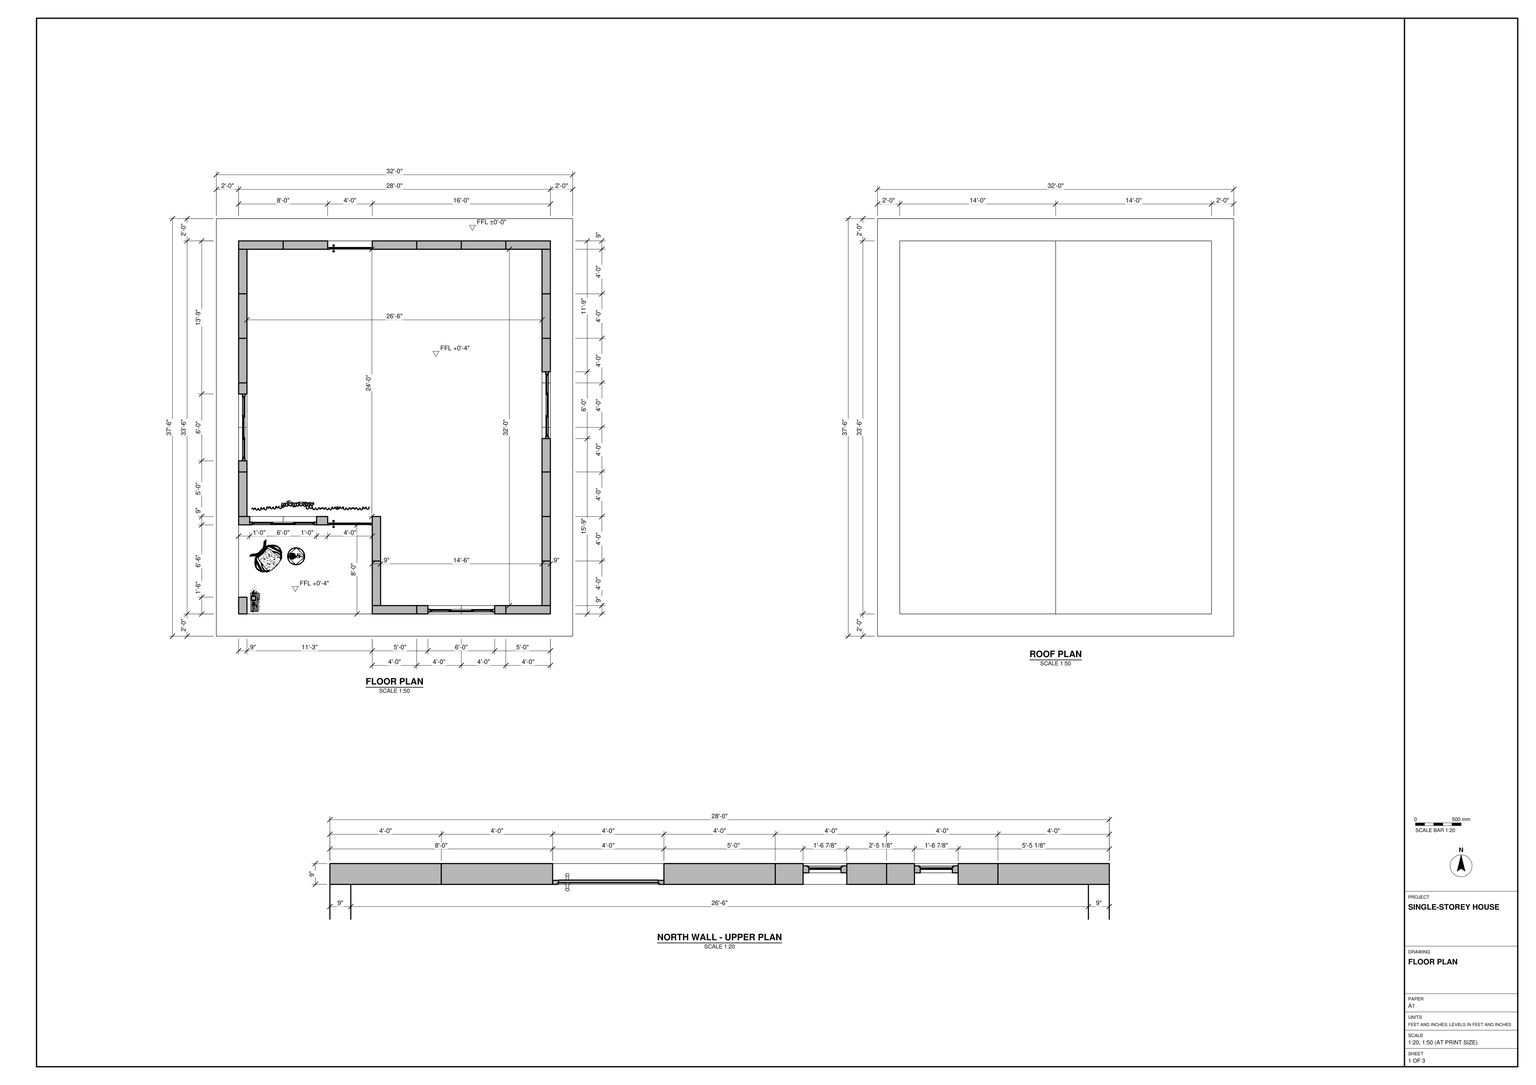
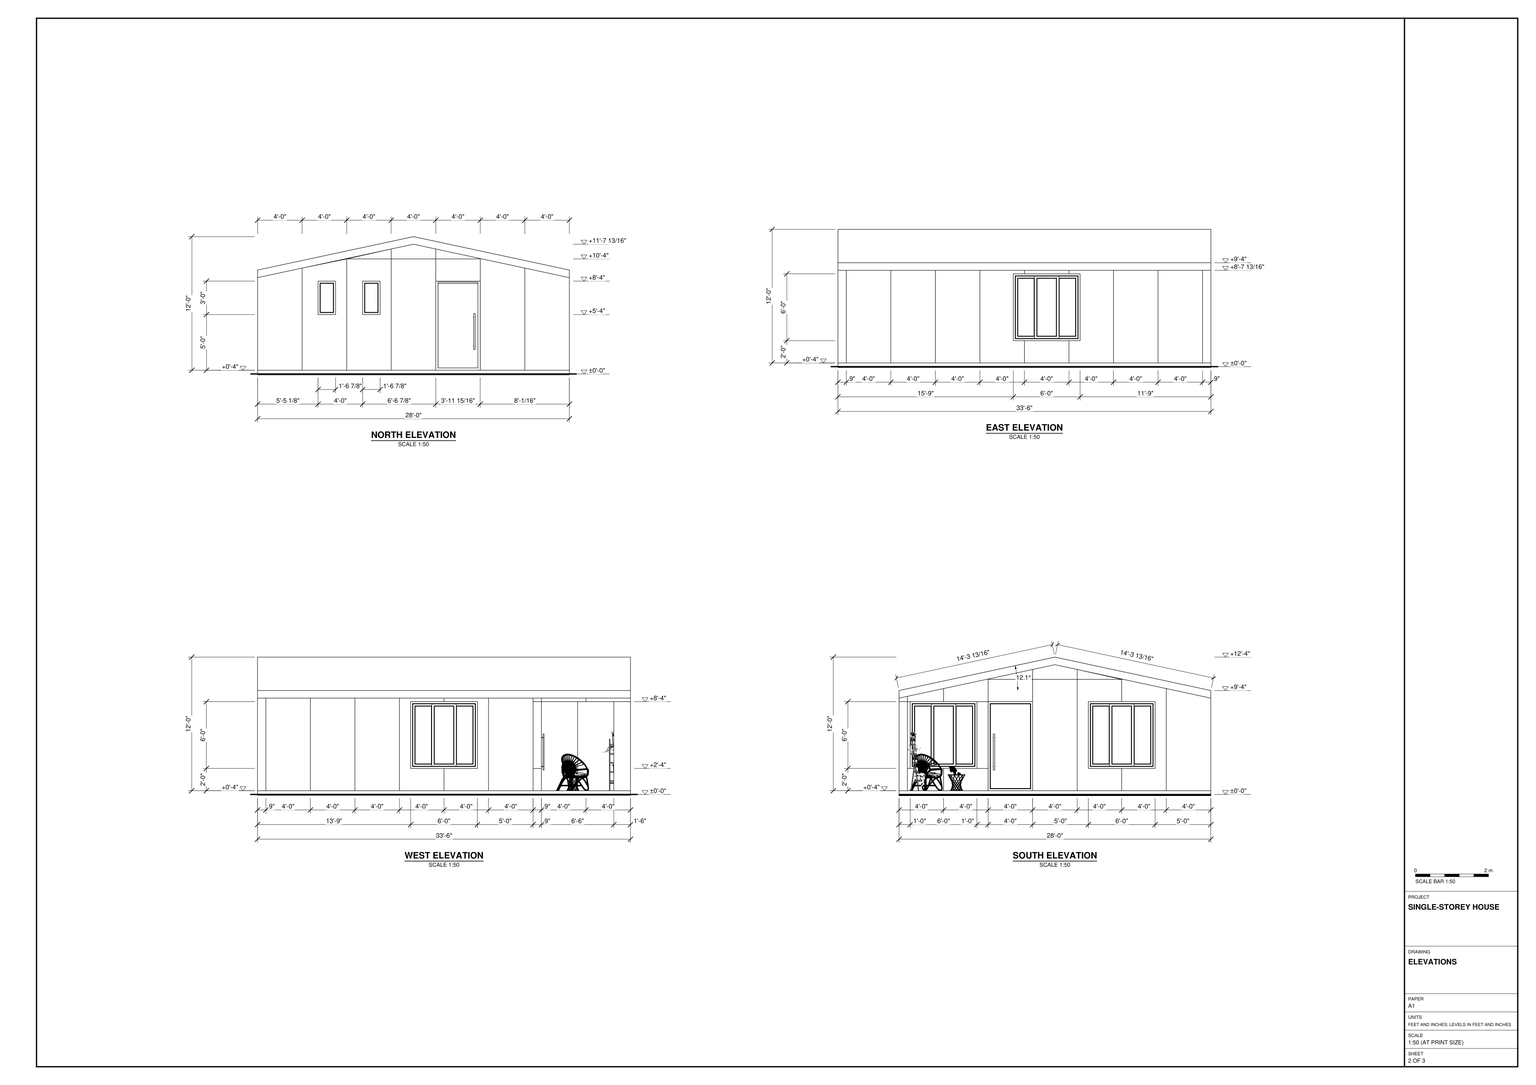
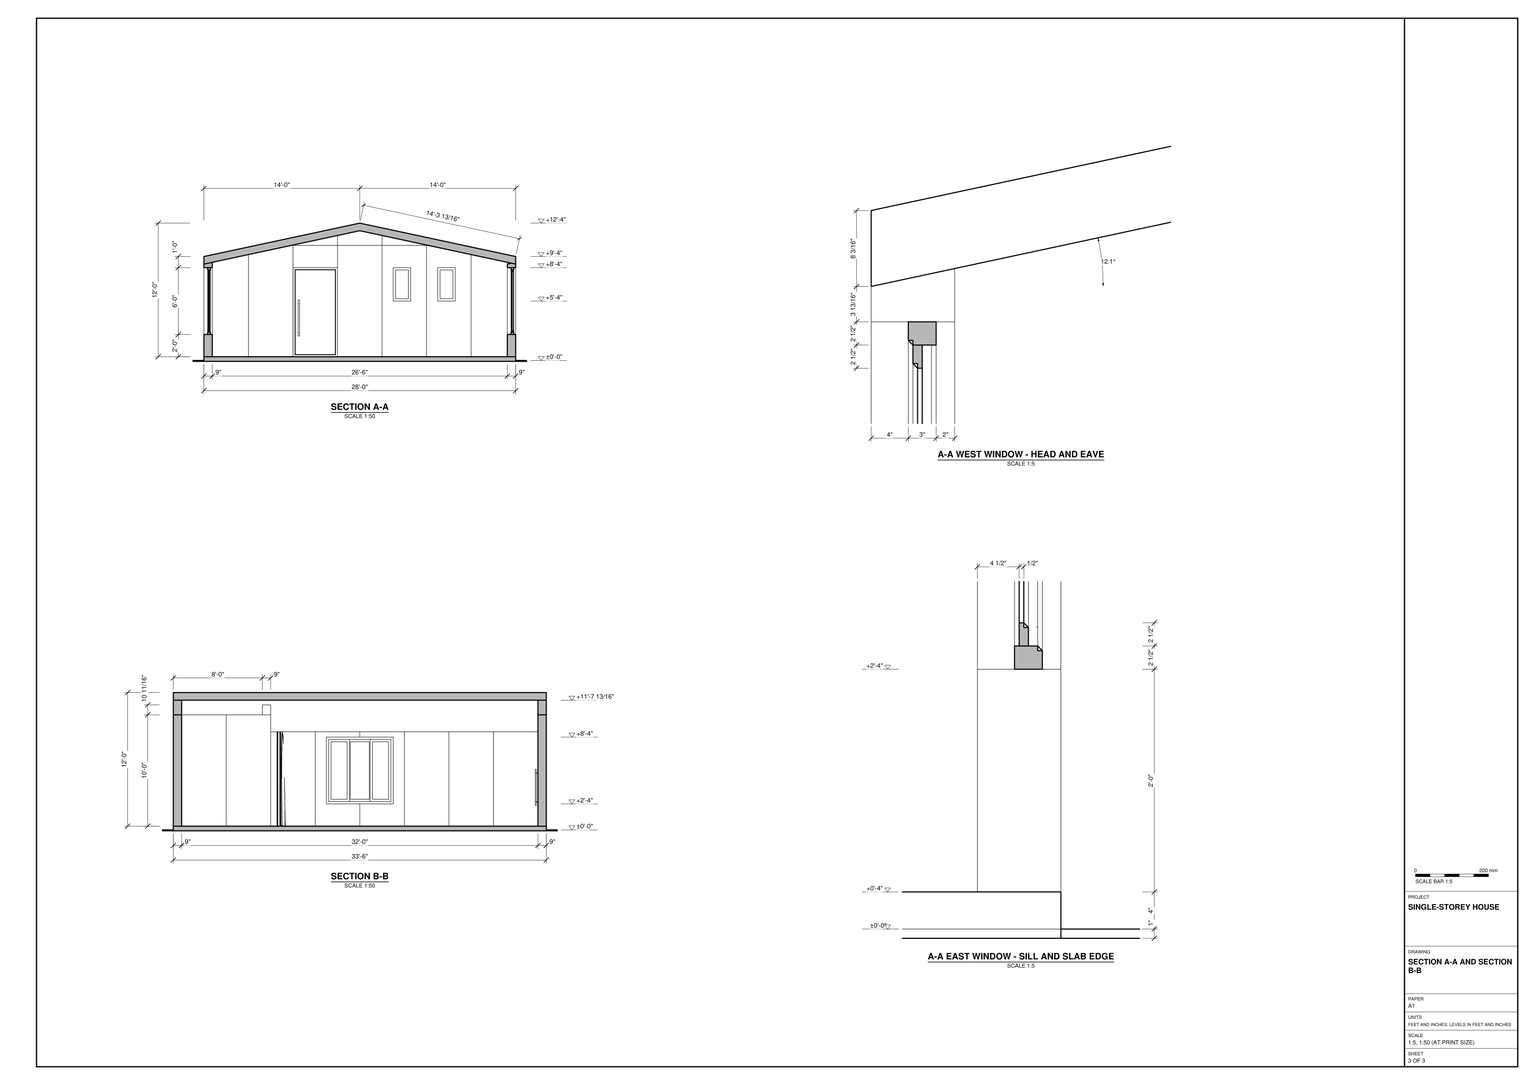
Build the house in SketchUp from task_files/diagram_01.pdf. Work in feet and inches. The complete model, including the surrounding ground, measures 128'-0" along X, 133'-6" along Y and 12'-5" along Z. Use ±0'-0" as the ground datum for the single storey. Set the finished floor and porch surface at +0'-4".

Set out the house within a 28'-0" by 33'-6" footprint. Follow the floor plan for the 9" walls, the open interior and the porch recessed into the southwest corner. Include the porch corner post and the seating and small table shown there. Model the slab edge and the vertical wall panel joints shown in the sections and elevations. Fit the north door beside the two narrow windows. On the south side, distinguish the door and window in the recessed wall from the window in the projecting wall. Use the sections to set the window frames, heads and sills into the side walls.

Carry the gable roof across the porch, with equal slopes meeting at a north–south ridge. Keep walls, slab, roof and each furniture or joinery piece in separate groups or components, and use components for repeated parts. Decor and loose items may be any suitable library components, for example from 3D Warehouse. Save one SketchUp model as output_files/single_storey_gabled_house_with_a_recessed_porch.skp.

# SketchUp Ruby script. Lengths in inches.
U = 1.inch
M = Sketchup.active_model
def pt(a) = Geom::Point3d.new(a.map { |v| v * U })
def face(e, loops, mat)
  f = e.add_face(loops[0].map { |a| pt(a) })
  loops[1..].each { |l| e.add_face(l.map { |a| pt(a) }).erase! }
  f.material = f.back_material = mat if mat
  f
end
# faces: each face lists its corners as indices into pts; further lists are holes
def faces(e, pts, list, mat = nil) = list.each { |f| face(e, (f[0].is_a?(Array) ? f : [f]).map { |l| l.map { |i| pts[i] } }, mat) }
# xy, xz, yz: faces in a plane at the given z, y or x. An outline is a flat list of corners, or four numbers for a rectangle; further outlines are holes
def ring(l) = l.size == 4 ? [[l[0], l[1]], [l[2], l[1]], [l[2], l[3]], [l[0], l[3]]] : l.each_slice(2).to_a
def flat(e, list, mat, &to3) = list.each { |f| face(e, (f[0].is_a?(Array) ? f : [f]).map { |l| ring(l).map { |u, v| to3.(u, v) } }, mat) }
def xy(e, z, list, mat = nil) = flat(e, list, mat) { |x, y| [x, y, z] }
def xz(e, y, list, mat = nil) = flat(e, list, mat) { |x, z| [x, y, z] }
def yz(e, x, list, mat = nil) = flat(e, list, mat) { |y, z| [x, y, z] }
def lines(e, pts, list) = list.each { |a, b| e.add_line(pt(pts[a]), pt(pts[b])) }
# prism: a flat outline (further loops are holes) pulled along v
def prism(e, loops, v, mat = nil)
  f = face(e, loops, mat); d = Geom::Vector3d.new(v.map { |x| x * U })
  f.pushpull(f.normal.samedirection?(d) ? d.length : -d.length)
end
def box(e, o, s, mat = nil) = prism(e, [[o, [o[0] + s[0], o[1], o[2]], [o[0] + s[0], o[1] + s[1], o[2]], [o[0], o[1] + s[1], o[2]]]], [0, 0, s[2]], mat)
def at(x, y, z, deg = 0) = Geom::Transformation.translation(pt([x, y, z])) * Geom::Transformation.rotation(ORIGIN, Z_AXIS, deg.degrees)
def axes(o, x, y, z) = Geom::Transformation.new([*x, 0, *y, 0, *z, 0, *pt(o).to_a, 1])
def part(name) = M.definitions.add(name)
# library, detail: a bought-in or finely detailed component or shape, given as its bounding box
def library(name, o, s) = part(name).tap { |d| box(d.entities, o, s) }
def detail(e, o, s) = box(e.add_group.entities, o, s)
def put(e, d, t, mat = nil) = e.add_instance(d, t).tap { |i| i.material = mat if mat }
def group(e, t, mat = nil) = e.add_group.tap { |g| g.transformation = t; g.material = mat if mat }.entities
root = M.entities
M.materials.add("Grass 02").color = [100, 122, 63]
M.materials.add("Marble 05_1").color = [239, 239, 239]
M.materials.add("Shingle 02").color = [69, 69, 69]
M.materials.add("Stone 01, Wall").color = [117, 118, 120]
M.materials.add("Wood 09_ Planks2").color = [153, 135, 119]
M.materials.add("[0135_DarkGray]1").color = [53, 53, 53]
M.materials.add("[Color M00]2").color = [53, 53, 53]
M.materials.add("[Translucent_Glass_Blue]").color = [0, 0, 0]
M.materials["[Translucent_Glass_Blue]"].alpha = 0.15
c1 = part("Exterior wall panel \#4")
prism(c1.entities,[[[0,0,0],[0,0,99.82],[0,48,110.1],[0,48,0]]],[9,0,0])
c2 = part("Exterior wall panel \#3")
prism(c2.entities,[[[9,0,0],[9,48,0],[9,48,120.39],[9,46.18,120],[9,0,110.1]]],[-9,0,0])
c3 = part("Short wall panel")
box(c3.entities,[0,0,96],[9,48,24])
c4 = part("Exterior wall panel \#1")
box(c4.entities,[0,0,0],[9,48,120])
c5 = part("Window opening panel \#1")
prism(c5.entities,[[[0,0,0],[0,0,120],[0,48,110.1],[0,48,0]],[[0,12,60],[0,30.85,60],[0,30.85,96],[0,12,96]]],[9,0,0])
c6 = part("Exterior wall panel \#5")
prism(c6.entities,[[[0,0,0],[0,0,110.1],[0,48,99.82],[0,48,0]]],[9,0,0])
c7 = part("Window opening panel \#2")
prism(c7.entities,[[[0,48,0],[0,0,0],[0,0,120],[0,48,120]],[[0,12,60],[0,30.85,60],[0,30.85,96],[0,12,96]]],[9,0,0])
c8 = part("Exterior wall panel")
prism(c8.entities,[[[9,48,0],[0,48,0],[0,48,101.75],[9,48,99.82]]],[0,-48,0])
c9 = part("Notched wall panel")
xy(c9.entities,0,[[0,0,9,48]])
xy(c9.entities,24,[[0,0,9,12]])
xy(c9.entities,96,[[0,0,9,12]])
xz(c9.entities,0,[[0,0,9,24],[0,96,9,96,9,99.82,4.5,100.78,0,99.82]])
xz(c9.entities,12,[[0,24,9,96]])
xz(c9.entities,48,[[0,0,0,99.82,4.5,100.78,9,99.82,9,0]])
yz(c9.entities,0,[[0,0,0,24,12,24,12,96,0,96,0,99.82,48,99.82,48,0]])
yz(c9.entities,9,[[0,0,48,0,48,99.82,0,99.82,0,96,12,96,12,24,0,24]])
p = [[4.5,0,100.78],[4.5,48,100.78],[0,48,99.82],[0,0,99.82],[9,0,99.82],[9,48,99.82]]
faces(c9.entities,p,[[0,1,2,3],[0,4,5,1]])
c10 = part("Short wall panel \#1")
box(c10.entities,[0,0,0],[48,9,24])
c11 = part("Wall infill strip")
prism(c11.entities,[[[0,9,0],[0,0,0],[0,0,5.75],[0,9,3.82]]],[48,0,0])
c12 = part("Exterior wall panel \#6")
prism(c12.entities,[[[0,0,0],[0,0,99.82],[0,48,110.1],[0,48,0]]],[9,0,0])
c13 = part("Window opening panel")
prism(c13.entities,[[[9,48,0],[9,48,24],[9,12,24],[9,12,96],[9,48,96],[9,48,120],[9,46.18,120],[9,0,110.1],[9,0,0]]],[-9,0,0])
c14 = part("Window opening panel \#3")
prism(c14.entities,[[[0,48,0],[0,0,0],[0,0,120],[0,48,120],[0,48,96],[0,12,96],[0,12,24],[0,48,24]]],[9,0,0])
c15 = part("Short wall panel \#2")
box(c15.entities,[0,0,96],[9,48,24])
c16 = part("Sloped wall panel")
prism(c16.entities,[[[0,48,96],[0,0,96],[0,0,110.1],[0,46.18,120],[0,48,120.39]]],[9,0,0])
c17 = part("Sloped wall panel \#1")
prism(c17.entities,[[[0,48,96],[0,0,96],[0,0,99.82],[0,9,101.75],[0,48,110.1]]],[9,0,0])
c18 = part("Exterior wall panel \#2")
prism(c18.entities,[[[0,0,0],[9,0,0],[9,0,99.82],[0,0,101.75]]],[0,48,0])
c19 = part("Window pane")
box(c19.entities,[0,0,0],[17.33,0.5,62])
c20 = part("Window sash")
xy(c20.entities,0,[[0,0,22.33,1]])
xy(c20.entities,2,[[2,0,20.33,0.5]])
xy(c20.entities,2.5,[[2.5,0.5,19.83,1]])
xy(c20.entities,64.5,[[2.5,0.5,19.83,1]])
xy(c20.entities,65,[[2,0,20.33,0.5]])
xy(c20.entities,67,[[0,0,22.33,1]])
xz(c20.entities,0,[[[0,0,22.33,67],[2,2,20.33,65]]])
xz(c20.entities,0.5,[[[2,2,20.33,65],[2.5,2.5,19.83,64.5]]])
xz(c20.entities,1,[[[0,0,22.33,67],[2.5,2.5,19.83,64.5]]])
yz(c20.entities,0,[[0,0,1,67]])
yz(c20.entities,2,[[0,2,0.5,65]])
yz(c20.entities,2.5,[[0.5,2.5,1,64.5]])
yz(c20.entities,19.83,[[0.5,2.5,1,64.5]])
yz(c20.entities,20.33,[[0,2,0.5,65]])
yz(c20.entities,22.33,[[0,0,1,67]])
p = [[20.33,0,2],[19.83,0.5,2.5],[2.5,0.5,2.5],[2,0,2],[2.5,0.5,64.5],[2,0,65],
  [20.33,0,65],[19.83,0.5,64.5]]
faces(c20.entities,p,[[0,1,2,3],[4,5,3,2],[6,7,1,0],[7,6,5,4]])
put(c20.entities,c19,at(2.5,0.5,2.5),"[Translucent_Glass_Blue]")
c21 = part("Window frame")
xy(c21.entities,0,[[0,0,72,3]])
xy(c21.entities,2,[[2,0,70,0.5]])
xy(c21.entities,2.5,[[2.5,0.5,69.5,3]])
xy(c21.entities,69.5,[[2.5,0.5,69.5,3]])
xy(c21.entities,70,[[2,0,70,0.5]])
xy(c21.entities,72,[[0,0,72,3]])
xz(c21.entities,0,[[[0,0,72,72],[2,2,70,70]]])
xz(c21.entities,0.5,[[[2,2,70,70],[2.5,2.5,69.5,69.5]]])
xz(c21.entities,3,[[[0,0,72,72],[2.5,2.5,69.5,69.5]]])
yz(c21.entities,0,[[0,0,3,72]])
yz(c21.entities,2,[[0,2,0.5,70]])
yz(c21.entities,2.5,[[0.5,2.5,3,69.5]])
yz(c21.entities,69.5,[[0.5,2.5,3,69.5]])
yz(c21.entities,70,[[0,2,0.5,70]])
yz(c21.entities,72,[[0,0,3,72]])
p = [[70,0,2],[69.5,0.5,2.5],[2.5,0.5,2.5],[2,0,2],[2.5,0.5,69.5],[2,0,70],
  [70,0,70],[69.5,0.5,69.5]]
faces(c21.entities,p,[[0,1,2,3],[4,5,3,2],[6,7,1,0],[5,4,7,6]])
c22 = part("Triple panel window \#1")
put(c22.entities,c20,axes([261.3,0.5,26.53],[1.1791,0,0],[0,1,0],[0,0,1]),"[0135_DarkGray]1")
put(c22.entities,c21,at(238.46,0,24.03),"[0135_DarkGray]1")
put(c22.entities,c20,at(285.63,1.5,26.53),"[0135_DarkGray]1")
put(c22.entities,c20,at(240.96,1.5,26.53),"[0135_DarkGray]1")
c23 = part("Triple panel window")
put(c23.entities,c20,axes([261.3,0.5,26.53],[1.1791,0,0],[0,1,0],[0,0,1]),"[0135_DarkGray]1")
put(c23.entities,c21,at(238.46,0,24.03),"[0135_DarkGray]1")
put(c23.entities,c20,at(285.63,1.5,26.53),"[0135_DarkGray]1")
put(c23.entities,c20,at(240.96,1.5,26.53),"[0135_DarkGray]1")
c24 = part("Wall pier")
box(c24.entities,[0,0,0],[12,9,72])
c25 = part("Component\#19")
box(c25.entities,[0,0,0],[9,18,96])
c26 = part("Component\#27")
prism(c26.entities,[[[9,0,96],[9,0,101.75],[0,0,99.82],[0,0,96]]],[0,48,0])
c27 = part("Component\#20")
prism(c27.entities,[[[9,0,96],[9,0,101.75],[0,0,99.82],[0,0,96]]],[0,48,0])
c28 = part("Single panel window")
xy(c28.entities,0,[[0,6,18.85,9]])
xy(c28.entities,2,[[2,8.5,16.85,9]])
xy(c28.entities,2.5,[[2.5,6,16.35,8.5]])
xy(c28.entities,33.5,[[2.5,6,16.35,8.5]])
xy(c28.entities,34,[[2,8.5,16.85,9]])
xy(c28.entities,36,[[0,6,18.85,9]])
xz(c28.entities,6,[[[0,0,18.85,36],[2.5,2.5,16.35,33.5]]])
xz(c28.entities,8.5,[[[2,2,16.85,34],[2.5,2.5,16.35,33.5]]])
xz(c28.entities,9,[[[0,0,18.85,36],[2,2,16.85,34]]])
yz(c28.entities,0,[[6,0,9,36]])
yz(c28.entities,2,[[8.5,2,9,34]])
yz(c28.entities,2.5,[[6,2.5,8.5,33.5]])
yz(c28.entities,16.35,[[6,2.5,8.5,33.5]])
yz(c28.entities,16.85,[[8.5,2,9,34]])
yz(c28.entities,18.85,[[6,0,9,36]])
p = [[2,9,2],[2.5,8.5,2.5],[16.35,8.5,2.5],[16.85,9,2],[2,9,34],[2.5,8.5,33.5],
  [16.35,8.5,33.5],[16.85,9,34]]
faces(c28.entities,p,[[0,1,2,3],[4,5,1,0],[6,7,3,2],[7,6,5,4]])
g1 = group(c28.entities,at(2.5,7.5,2.5),"[Translucent_Glass_Blue]")
box(g1,[0,0,0],[13.85,0.5,31])
c29 = part("OuterShell1")
xy(c29.entities,0,[[0,0,9,48]])
xy(c29.entities,24,[[0,0,9,36]])
xy(c29.entities,96,[[0,0,9,36]])
xz(c29.entities,0,[[0,0,9,24],[0,96,9,96,9,101.75,0,99.82]])
xz(c29.entities,36,[[0,24,9,96]])
xz(c29.entities,48,[[0,0,0,99.82,9,101.75,9,0]])
yz(c29.entities,0,[[0,0,0,24,36,24,36,96,0,96,0,99.82,48,99.82,48,0]])
yz(c29.entities,9,[[0,0,48,0,48,101.75,0,101.75,0,96,36,96,36,24,0,24]])
p = [[9,48,101.75],[0,48,99.82],[0,0,99.82],[9,0,101.75]]
faces(c29.entities,p,[[0,1,2,3]])
c30 = part("Gable infill panel \#2")
prism(c30.entities,[[[48,9,0],[0,9,0],[0,9,10.68]]],[0,-9,0])
c31 = part("Gable infill panel")
prism(c31.entities,[[[48,0,0],[48,0,10.68],[24,0,15.82],[0,0,10.68],[0,0,0]]],[0,9,0])
c32 = part("Gable infill panel \#1")
prism(c32.entities,[[[0,48,96],[0,0,96],[0,0,96.39],[0,48,106.68]]],[9,0,0])
c33 = library("BARN 550 done by",[0.96,0,0],[275.97,12.64,1])
c34 = part("Ground plane")
xy(c34.entities,0,[[[0,0,1536,1602],[600,600,936,1002]]])
xy(c34.entities,1,[[[0,0,1536,1602],[576,576,960,1026]]])
xy(c34.entities,1,[[[576,576,960,1026],[600,600,936,1002]]],"Grass 02")
xz(c34.entities,0,[[0,0,1536,1]])
xz(c34.entities,600,[[600,0,936,1]])
xz(c34.entities,1002,[[600,0,936,1]])
xz(c34.entities,1602,[[0,0,1536,1]])
yz(c34.entities,0,[[0,0,1602,1]])
yz(c34.entities,600,[[600,0,1002,1]])
yz(c34.entities,936,[[600,0,1002,1]])
yz(c34.entities,1536,[[0,0,1602,1]])
c35 = library("Group\#1",[0,0,0],[430.82,336,0.01])
c36 = library("Group\#59",[0,0,-2.5],[47.9375,7.6,96])
c37 = library("Group\#90",[14.45,1.85,0],[11.92,126.54,108.875])
c38 = library("Group\#100",[-8.55,-14.17,0],[162.72,113.29,102.57])
c39 = library("Group\#61",[20.28,-1.68,-0.15],[30.59,22.83,66.38])
c40 = part("Group\#4")
box(c40.entities,[0,0,0],[48,9,24])
c41 = library("Group\#23",[0,0,0],[69.84,168.55,64.8])
c42 = library("Group\#77",[0,0,0],[119.8,109.12,43.25])
p = [[936,600,0],[1208,600,0]]
lines(root,p,[[0,1]])
put(root,c1,at(600,1002,0,-90),"Wood 09_ Planks2")
put(root,c2,at(648,1002,0,-90),"Wood 09_ Planks2")
put(root,c3,at(696,1002,0,-90),"Wood 09_ Planks2")
put(root,c4,at(744,1002,0,-90),"Wood 09_ Planks2")
put(root,c5,at(840,1002,0,-90),"Wood 09_ Planks2")
put(root,c6,at(888,1002,0,-90),"Wood 09_ Planks2")
put(root,c7,at(792,1002,0,-90),"Wood 09_ Planks2")
put(root,c8,at(927,945,0),"Wood 09_ Planks2")
put(root,c8,at(927,897,0),"Wood 09_ Planks2")
put(root,c9,at(927,849,0),"Wood 09_ Planks2")
put(root,c9,at(936,801,0,180),"Wood 09_ Planks2")
put(root,c10,at(927,849,0,-90),"Wood 09_ Planks2")
put(root,c11,at(927,849,96,-90),"Wood 09_ Planks2")
put(root,c8,at(927,705,0),"Wood 09_ Planks2")
put(root,c8,at(927,657,0),"Wood 09_ Planks2")
put(root,c8,at(927,609,0),"Wood 09_ Planks2")
put(root,c12,at(936,600,0,90),"Wood 09_ Planks2")
put(root,c13,at(888,600,0,90),"Wood 09_ Planks2")
put(root,c14,axes([792,600,0],[0,1,0],[1,0,0],[0,0,1]),"Wood 09_ Planks2")
put(root,c4,at(792,600,0,90),"Wood 09_ Planks2")
put(root,c4,at(753,657,0,180),"Wood 09_ Planks2")
put(root,c4,at(753,705,0,180),"Wood 09_ Planks2")
put(root,c15,at(696,705,0,-90),"Wood 09_ Planks2")
put(root,c16,at(648,705,0,-90),"Wood 09_ Planks2")
put(root,c17,at(600,705,0,-90),"Wood 09_ Planks2")
put(root,c18,at(609,753,0,180),"Wood 09_ Planks2")
put(root,c18,at(609,897,0,180),"Wood 09_ Planks2")
put(root,c18,at(609,945,0,180),"Wood 09_ Planks2")
put(root,c18,at(609,993,0,180),"Wood 09_ Planks2")
put(root,c22,at(565.54,602,-0.03))
put(root,c23,at(934,550.54,-0.03,90))
put(root,c23,axes([604,526.54,-0.03],[0,1,0],[1,0,0],[0,0,1]))
put(root,c23,at(373.54,696,-0.03),"[0135_DarkGray]1")
put(root,c24,at(600,696,24),"Wood 09_ Planks2")
put(root,c24,at(684,696,24),"Wood 09_ Planks2")
put(root,c25,at(600,600,0),"Wood 09_ Planks2")
put(root,c26,at(600,648,0),"Wood 09_ Planks2")
put(root,c27,at(600,600,0),"Wood 09_ Planks2")
put(root,c28,at(804,992,60),"[0135_DarkGray]1")
put(root,c28,at(852,992,60),"[0135_DarkGray]1")
put(root,c29,at(600,801,0),"Wood 09_ Planks2")
put(root,c29,axes([600,801,0],[1,0,0],[0,-1,0],[0,0,1]),"Wood 09_ Planks2")
put(root,c30,at(792,600,120),"Wood 09_ Planks2")
put(root,c31,at(744,600,120),"Wood 09_ Planks2")
put(root,c30,at(792,993,120),"Wood 09_ Planks2")
put(root,c31,at(744,993,120),"Wood 09_ Planks2")
put(root,c32,at(696,1002,24,-90),"Wood 09_ Planks2")
put(root,c32,at(696,705,24,-90),"Wood 09_ Planks2")
put(root,c33,axes([988,600,-5],[1,0,0],[0,0,1],[0,-1,0]))
put(root,c34,at(0,0,-5),"Stone 01, Wall")
put(root,c35,at(600,1030.82,0,-90))
g2 = group(root,at(600,600,0),"Wood 09_ Planks2")
xy(g2,-5,[[0,0,336,402]])
xy(g2,0,[[0,0,336,402]],"Marble 05_1")
xz(g2,0,[[0,-5,336,0]])
xz(g2,402,[[0,-5,336,0]])
yz(g2,0,[[0,-5,402,0]])
yz(g2,336,[[0,-5,402,0]])
put(root,c36,at(696.0625,693.125,2.5))
put(root,c37,axes([612.25,695.84,-0.4],[0,1,0],[1,0,0],[0,0,0.93686]),"[Color M00]2")
put(root,c38,axes([611.77,644.89,0],[0.38707,0,0],[0,0.38707,0],[0,0,0.38707]))
put(root,c39,axes([629.14,650.74,0],[0,-1,0],[-1,0,0],[0,0,1]))
put(root,c36,at(696.0625,990.125,2.5))
g3 = group(root,at(600,600,99.82),"Shingle 02")
xz(g3,0,[[0,0,168,36,336,0,336,8.18,168,44.18,0,8.18]])
xz(g3,402,[[0,0,0,8.18,168,44.18,336,8.18,336,0,168,36]])
yz(g3,0,[[0,0,402,8.18]])
yz(g3,336,[[0,0,402,8.18]])
p = [[168,0,36],[0,0,0],[0,402,0],[168,402,36],[336,0,0],[336,402,0],
  [0,0,8.18],[168,0,44.18],[168,402,44.18],[0,402,8.18],[336,0,8.18],[336,402,8.18]]
faces(g3,p,[[0,1,2,3],[4,0,3,5]],"Wood 09_ Planks2")
faces(g3,p,[[6,7,8,9],[7,10,11,8]])
put(root,c40,at(600,696,0),"Wood 09_ Planks2")
put(root,c40,at(648,696,0),"Wood 09_ Planks2")
put(root,c41,at(931.77,570.49,-4,180))
put(root,c42,at(685.2,425.375,-4,90))
